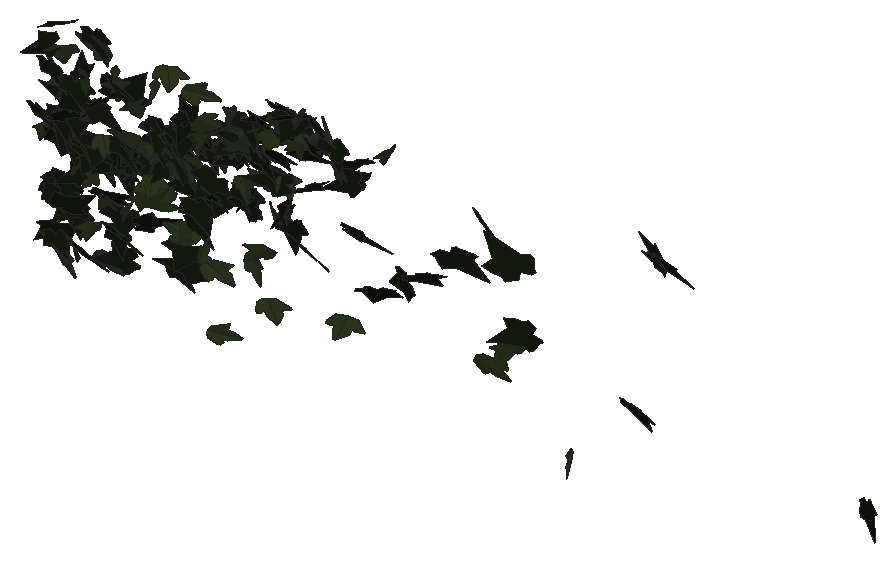
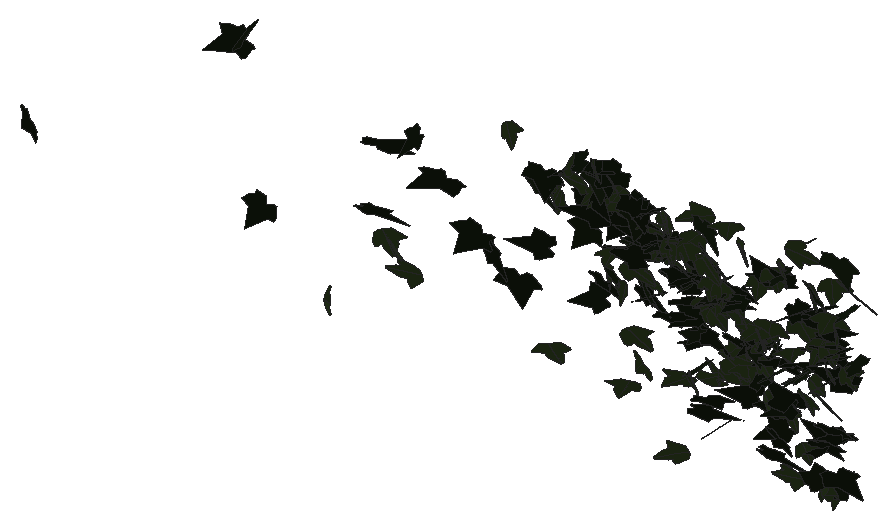
# SketchUp Ruby script. Lengths in millimetres.
U = 1.mm
M = Sketchup.active_model
def pt(a) = Geom::Point3d.new(a.map { |v| v * U })
def face(e, loops, mat)
  f = e.add_face(loops[0].map { |a| pt(a) })
  loops[1..].each { |l| e.add_face(l.map { |a| pt(a) }).erase! }
  f.material = f.back_material = mat if mat
  f
end
# faces: each face lists its corners as indices into pts; further lists are holes
def faces(e, pts, list, mat = nil) = list.each { |f| face(e, (f[0].is_a?(Array) ? f : [f]).map { |l| l.map { |i| pts[i] } }, mat) }
# xy, xz, yz: faces in a plane at the given z, y or x. An outline is a flat list of corners, or four numbers for a rectangle; further outlines are holes
def ring(l) = l.size == 4 ? [[l[0], l[1]], [l[2], l[1]], [l[2], l[3]], [l[0], l[3]]] : l.each_slice(2).to_a
def flat(e, list, mat, &to3) = list.each { |f| face(e, (f[0].is_a?(Array) ? f : [f]).map { |l| ring(l).map { |u, v| to3.(u, v) } }, mat) }
def xy(e, z, list, mat = nil) = flat(e, list, mat) { |x, y| [x, y, z] }
def xz(e, y, list, mat = nil) = flat(e, list, mat) { |x, z| [x, y, z] }
def yz(e, x, list, mat = nil) = flat(e, list, mat) { |y, z| [x, y, z] }
def lines(e, pts, list) = list.each { |a, b| e.add_line(pt(pts[a]), pt(pts[b])) }
# prism: a flat outline (further loops are holes) pulled along v
def prism(e, loops, v, mat = nil)
  f = face(e, loops, mat); d = Geom::Vector3d.new(v.map { |x| x * U })
  f.pushpull(f.normal.samedirection?(d) ? d.length : -d.length)
end
def box(e, o, s, mat = nil) = prism(e, [[o, [o[0] + s[0], o[1], o[2]], [o[0] + s[0], o[1] + s[1], o[2]], [o[0], o[1] + s[1], o[2]]]], [0, 0, s[2]], mat)
def at(x, y, z, deg = 0) = Geom::Transformation.translation(pt([x, y, z])) * Geom::Transformation.rotation(ORIGIN, Z_AXIS, deg.degrees)
def axes(o, x, y, z) = Geom::Transformation.new([*x, 0, *y, 0, *z, 0, *pt(o).to_a, 1])
def part(name) = M.definitions.add(name)
# library, detail: a bought-in or finely detailed component or shape, given as its bounding box
def library(name, o, s) = part(name).tap { |d| box(d.entities, o, s) }
def detail(e, o, s) = box(e.add_group.entities, o, s)
def put(e, d, t, mat = nil) = e.add_instance(d, t).tap { |i| i.material = mat if mat }
def group(e, t, mat = nil) = e.add_group.tap { |g| g.transformation = t; g.material = mat if mat }.entities
root = M.entities
M.materials.add("efeu1").color = [18, 25, 13]
M.materials.add("efeu2").color = [43, 57, 29]
c1 = part("ivyleaf_9")
p = [[39.1,54.8,31.7],[34.5,51.8,30.2],[-5.3,25.2,17.3],[-17.9,28.3,20.9],[-21.6,21.7,17],[-20.2,4.3,5.3],
  [-22.9,-0.3,2.5],[-17.1,-4,-0.6],[-2,-2.1,-1.2],[-0.7,-15.4,-10.1],[16.6,-22.3,-16.7],[21.1,-15.1,-12.5],
  [32.7,-10.7,-11],[46.1,-1.8,-6.6],[30.8,11.2,3.8]]
faces(c1.entities,p,[[0,1,2,3,4,5,6,7,8,9,10,11,12,13,14]],"efeu1")
c2 = part("ivyleaf_10")
p = [[0,12.8,-0.8],[-1.5,51.3,-10.9],[-4.9,51,-11.6],[-13.6,26.5,-7.3],[-13.2,15.9,-4.6],[-21.1,19.3,-7.2],
  [-29.5,16.3,-8.3],[-29.2,8.3,-6.2],[-19.7,-9.8,0.5],[-7.6,-13,4],[1,-12.2,5.8],[-0.4,51.1,-11.1],
  [-1.5,51.1,-10.9],[1,-12.4,5.9],[16.9,-12.4,3.5],[35.1,9.1,-5.1],[35,12.9,-6.1],[20.5,16.4,-4.9],
  [15.8,15,-3.8],[15.3,27.6,-7.1],[12.8,31.3,-7.8]]
faces(c2.entities,p,[[0,1,2,3,4,5,6,7,8,9,10],[11,12,0,13,14,15,16,17,18,19,20]],"efeu2")
put(root,c1,axes([4895,793.5,3135.5],[0.99985,-0.9512,0.16756],[0.29482,-0.10529,-1.0834],[1.81439,0.54128,0.08371]))
put(root,c1,axes([4961.3,784.3,3378.4],[-1.89203,0.5811,-0.0485],[-0.01971,-0.11345,-1.14688],[-1.10962,-0.98882,0.10308]))
put(root,c2,axes([4943.9,791.7,3096.3],[-0.58928,-1.00709,0.34545],[-0.09077,-0.34628,-1.05226],[2.02429,-0.3087,0.05338]))
put(root,c1,axes([4962.2,812,2755.9],[0.28697,0.52098,-0.9616],[-0.43571,-0.93416,-0.54201],[-2.03534,0.27343,-0.01955]))
put(root,c1,axes([4936.5,795.6,3298.9],[0.65973,-1.08228,0.0317],[0.04767,-0.02526,-1.13632],[2.06013,0.34717,0.01614]))
put(root,c1,axes([4984,780.5,3453.5],[0.3733,1.12783,0.06991],[-0.59622,0.12245,-1.09646],[-2.0663,0.16842,0.32901]))
put(root,c1,axes([4958.4,817.5,2889],[-0.64539,-0.93685,-0.37561],[0.2059,0.36022,-0.99614],[1.90991,-0.35541,-0.01953]))
put(root,c1,axes([4941.9,793.4,2697.1],[0.69518,-0.70686,0.73199],[0.65781,-0.6453,-0.79562],[1.82152,0.50281,0.00796]))
put(root,c1,axes([4980.3,824.5,2911.1],[-1.71841,-0.38438,-0.40311],[0.74559,0.10755,-0.98002],[0.75356,-0.98294,0.05041]))
put(root,c2,axes([4982.3,797.2,3233.2],[0.53522,-1.08965,-0.1569],[0.25302,0.19437,-1.11157],[2.07987,0.25676,0.1756]))
put(root,c1,axes([4971.6,788.7,2733.6],[0.1042,-1.05035,-0.32712],[-0.09159,0.32492,-1.05136],[2.09173,0.06655,-0.02974]))
put(root,c1,axes([4941.5,788.9,3060],[0.93088,-0.27009,1.00515],[1.82838,-0.31014,-0.55082],[0.76211,1.07395,0.09372]))
put(root,c1,axes([4973.9,806.5,2878.5],[-0.40069,-1.03674,-0.42166],[0.28163,0.3995,-1.05615],[2.11137,-0.25004,0.06086]))
put(root,c2,axes([5001.1,790.1,3373.3],[-1.33311,-0.90194,-0.06794],[0.08726,0.05042,-1.14198],[1.71922,-0.70194,0.00528]))
put(root,c1,axes([4984.2,793.4,3148],[-0.16469,-1.11858,-0.01331],[-0.00191,0.01343,-1.12192],[2.12903,-0.08651,-0.00204]))
put(root,c2,axes([5007.7,802.8,3161.3],[-0.77688,-1.01331,0.20273],[-0.05131,-0.20746,-1.09122],[1.96609,-0.40581,0.05163]))
put(root,c1,axes([5022.8,818.9,2843],[-1.89321,-0.32974,-0.01532],[0.03036,0.00056,-1.04797],[0.62751,-0.99487,0.00448]))
put(root,c1,axes([4986.9,795,3063.1],[0.94548,-0.73023,-0.66735],[-0.30899,0.67647,-0.86106],[1.85719,0.4843,0.19649]))
put(root,c2,axes([5002.2,797.2,3260.7],[-1.79745,-0.54668,-0.30729],[0.68518,-0.01779,-1.07486],[0.97727,-0.99301,0.18842]))
put(root,c1,axes([5006.1,801.2,3119.2],[-0.90927,-0.95182,0.29186],[-0.12886,-0.29191,-1.06282],[1.89036,-0.47772,0.06794]))
put(root,c1,axes([5026.2,779.8,3169.2],[0.02648,0.89594,-0.78841],[-0.03884,-0.78817,-0.89602],[-2.27102,0.02393,0.00613]))
put(root,c1,axes([5053.2,790.9,3201.9],[-0.25436,0.07532,1.12914],[-1.96334,0.45932,-0.15274],[-0.88544,-1.04012,0.01432]))
put(root,c2,axes([4993.1,793.4,2670.3],[-0.88924,0.53618,-0.86189],[0.95164,-0.70413,-0.7091],[-1.6812,-0.68217,0.05449]))
put(root,c2,axes([5004.3,805.8,3090.8],[1.11525,-0.64936,0.67422],[0.87348,-0.49395,-0.87464],[1.55271,0.74428,0.00776]))
put(root,c2,axes([5003.3,828.6,2686.1],[-0.60815,0.0155,1.03507],[1.43712,-0.73751,0.24415],[1.34769,0.79345,0.20672]))
put(root,c1,axes([5019.3,817.6,2824.3],[-0.42925,-1.06641,-0.15585],[0.10628,0.14745,-1.08973],[2.04839,-0.23112,0.02388]))
put(root,c1,axes([5004.6,781.2,2843.8],[-0.41443,-0.0664,1.09538],[2.07818,0.09809,0.22302],[-0.20797,1.1125,0.04572]))
put(root,c2,axes([5031.2,801.3,3163.3],[-1.16912,-0.93142,-0.56717],[0.59728,0.47243,-1.11575],[1.98767,-0.68981,0.00168]))
put(root,c1,axes([5026.2,812.1,3162.6],[-0.82502,-0.98611,-0.23385],[0.30034,0.18556,-1.07502],[1.90528,-0.45625,0.0682]))
put(root,c1,axes([5023.1,804.4,3069.5],[-0.26273,-1.06103,0.24216],[0.04039,-0.24668,-1.06873],[2.07088,-0.1298,0.05157]))
put(root,c1,axes([5070.2,783.6,2980.5],[-1.66615,0.62673,-0.08734],[0.13592,-0.05029,-1.07666],[-1.19662,-0.87836,-0.00068]))
put(root,c1,axes([5064.8,784.5,3307.3],[0.54372,0.31735,1.06051],[-0.12853,1.09821,-0.31044],[-2.10287,0.01493,0.29318]))
put(root,c1,axes([5047.7,789.7,3274.2],[-0.25318,-1.1131,-0.11797],[0.07277,0.11421,-1.12076],[2.12908,-0.13627,0.02428]))
put(root,c2,axes([5066.7,794.7,3022],[0.05634,-0.93695,0.58434],[0.07367,-0.58331,-0.93726],[2.10027,0.0456,0.0172]))
put(root,c1,axes([5028.4,805,2710.6],[1.3556,-0.62619,0.52452],[0.79045,-0.32162,-0.94796],[1.33866,0.82402,0.0286]))
put(root,c2,axes([5083.4,810.5,2975.3],[1.64045,-0.67832,-0.05307],[-0.08159,0.03133,-1.09684],[1.29236,0.863,-0.00189]))
put(root,c2,axes([5090.5,806.5,2800.7],[-0.74678,-0.94995,0.21409],[0.04261,-0.23956,-1.02191],[1.85279,-0.37737,0.10979]))
put(root,c2,axes([5113.5,796.5,3199.1],[-1.82115,-0.23761,0.53048],[-0.94755,-0.19228,-0.9842],[0.57092,-1.07706,0.05867]))
put(root,c2,axes([5099.6,766.1,3311.6],[0.96397,-0.78962,-0.6812],[-0.38347,0.66893,-0.92521],[1.94735,0.5226,0.15501]))
put(root,c1,axes([5092.1,812.2,3041.7],[-1.05486,-0.86571,0.42191],[-0.01281,-0.4833,-1.00052],[1.83283,-0.50163,0.23583]))
put(root,c1,axes([5080.1,812.5,3050.9],[0.96719,-0.94563,-0.21102],[-0.05406,0.22365,-1.0706],[1.8432,0.50277,0.07933]))
put(root,c1,axes([5108.5,821.3,3081.5],[-1.12385,-0.92501,0.03891],[0.1291,-0.08926,-1.09238],[1.75731,-0.58502,0.10514]))
put(root,c2,axes([5157.6,775.7,3425.3],[-0.14861,0.19579,-1.25186],[-2.04329,0.6559,0.16955],[1.28076,1.06913,0.12524]))
put(root,c1,axes([5139.8,786.8,3247.2],[-0.60774,0.78246,-0.78278],[0.48804,-0.74024,-0.84454],[-2.04913,-0.40837,0.03101]))
put(root,c1,axes([5105.8,825.1,3034.4],[0.46372,-1.06443,-0.00225],[0.00259,0.00262,-1.09196],[2.02583,0.24365,0.00191]))
put(root,c2,axes([5154.9,801.7,2900.8],[-1.54255,0.36473,0.68855],[-1.22178,0.2505,-0.88836],[-0.84045,-1.03357,0.02767]))
put(root,c1,axes([5116.1,786.6,3463.7],[0.23777,-1.14106,-0.07944],[0.03311,0.0818,-1.14758],[2.17666,0.1234,0.02613]))
put(root,c2,axes([5115.1,820.2,2697.9],[-0.83524,0.21107,-0.95915],[1.61639,-0.44597,-0.48674],[-0.93858,-0.95587,0.0153]))
put(root,c2,axes([5139.2,802.4,3106.4],[1.08697,0.9593,-0.02444],[-0.00142,-0.028,-1.11636],[-1.82634,0.57097,-0.01368]))
put(root,c1,axes([5128.1,771.4,3228.5],[0.85114,-0.84391,-0.60624],[0.07189,0.67278,-0.90866],[1.97629,0.33898,0.29415]))
put(root,c1,axes([5137.4,806.3,2918.9],[1.84182,-0.43318,0.00169],[0.08158,0.09165,-1.05544],[0.82038,0.9634,0.10116]))
put(root,c1,axes([5191.7,810.3,3059.6],[-2.03846,-0.19623,0.0523],[-0.10171,0.00146,-1.08884],[0.37289,-1.07234,-0.01106]))
put(root,c1,axes([5138.6,798.7,2921.4],[1.97474,0.33957,-0.26038],[0.47235,0.07878,1.09174],[0.66341,-1.06686,-0.00226]))
put(root,c1,axes([5177.7,821,2808.6],[-1.12659,-0.05492,-0.90653],[1.72743,-0.07337,-0.58823],[-0.06005,-1.08019,0.08604]))
put(root,c1,axes([5235.5,806.3,2736],[-1.83187,0.14666,0.53247],[-0.99706,0.09627,-0.97353],[-0.33278,-1.09577,-0.01426]))
put(root,c2,axes([5200.1,782.1,3358.7],[0.86246,-1.05296,-0.13502],[-0.02913,0.14031,-1.1456],[2.0202,0.45155,0.04112]))
put(root,c1,axes([5175.1,788.6,2830.5],[2.09998,-0.41949,-0.02096],[-0.03264,0.01385,-1.18043],[0.7987,1.10351,0.00685]))
put(root,c1,axes([5191.8,828.6,3016.8],[0.07398,-1.05919,0.23083],[0.11598,-0.22848,-1.05866],[2.0599,0.0509,0.05132]))
put(root,c1,axes([5246,776.7,3092.5],[-0.69455,0.91856,0.47704],[-0.66894,0.36579,-0.97322],[-1.85285,-0.47639,0.17255]))
put(root,c1,axes([5209.2,824.3,3056.2],[-0.91054,-0.97823,-0.09877],[0.09304,0.08604,-1.08894],[1.86893,-0.48088,0.00609]))
put(root,c2,axes([5225.3,786,3331.6],[-1.33233,-0.875,0.19659],[-0.02938,-0.2376,-1.11249],[1.70655,-0.68721,0.13433]))
put(root,c1,axes([5187.9,788.7,3337],[1.14529,-0.96735,-0.0528],[0.16998,0.11728,-1.1309],[1.83594,0.59259,0.13764]))
put(root,c1,axes([5212.8,811.5,3062],[-0.30557,-0.42356,1.01444],[-0.41974,-0.99195,-0.44908],[2.04968,-0.26628,0.05927]))
put(root,c1,axes([5219.8,801.1,2893.8],[-1.49126,-0.6028,-0.38934],[0.56572,0.25205,-0.98845],[1.24307,-0.83786,-0.01723]))
put(root,c2,axes([5229.1,799.6,3157.5],[-2.13061,-0.11384,0.02211],[-0.04337,0.00557,-1.12523],[0.21641,-1.11969,-0.00785]))
put(root,c2,axes([5238.1,819.3,3040],[-0.31358,-1.04964,0.22877],[-0.14572,-0.21938,-1.06171],[2.03937,-0.17707,-0.04069]))
put(root,c2,axes([5232.8,804,2918.1],[0.31779,-1.06075,0.22936],[0.16519,-0.21826,-1.07261],[2.05885,0.18124,0.05066]))
put(root,c1,axes([5216.2,798.1,3125],[0.09227,-1.10628,-0.13717],[0.12569,0.13991,-1.10503],[2.11787,0.0399,0.07156]))
put(root,c1,axes([5227.9,777.2,3296.9],[-1.49566,0.1479,1.03636],[1.94161,-0.18248,0.79964],[0.4469,1.28776,-0.00571]))
put(root,c2,axes([5252.9,816.6,3130.1],[0.7245,-1.03113,0.1237],[0.09716,-0.11301,-1.09912],[1.97414,0.38398,0.0087]))
put(root,c1,axes([5235.6,815.8,3097.3],[0.03295,-0.82058,0.74143],[0.28341,-0.73304,-0.81477],[2.08563,0.11258,0.099]))
put(root,c1,axes([5274.8,824.6,3071.4],[-1.34824,0.4181,-0.72129],[0.76287,-0.65913,-0.77575],[-1.39128,-0.76658,0.27362]))
put(root,c1,axes([5242.8,820.2,2966.5],[-0.11197,-0.52167,0.94009],[0.44356,-0.9253,-0.49888],[1.99754,0.17622,0.16347]))
put(root,c2,axes([5268.7,811.6,3082.4],[-0.03452,0.91133,-0.57721],[-0.45718,-0.5662,-0.88641],[-2.00151,0.11361,0.21242]))
put(root,c2,axes([5279.3,782.9,3286.8],[-1.05418,-0.94917,-0.30611],[0.27077,0.27137,-1.09888],[1.87867,-0.57172,-0.01339]))
put(root,c2,axes([5263.2,816.1,3136.4],[-1.83112,-0.21167,-0.50134],[1.02747,-0.24304,-0.93344],[0.1304,-1.05734,0.31492]))
put(root,c1,axes([5266.3,795.7,3088.1],[0.15876,-0.73778,-0.80673],[0.11525,0.81095,-0.73538],[2.07744,0.01139,0.10245]))
put(root,c2,axes([5297.2,815,2999.3],[1.30859,0.80245,-0.16364],[-0.23494,-0.10968,-1.0565],[-1.54085,0.69822,0.02211]))
put(root,c2,axes([5310.1,786.4,2985.1],[-0.88043,-0.96244,0.09659],[-0.04227,-0.09647,-1.06762],[1.84043,-0.46263,0.02168]))
put(root,c2,axes([5319.4,807.9,3090],[0.62326,-1.02109,-0.106],[0.06065,0.12132,-1.07022],[1.95284,0.32212,0.06707]))
put(root,c1,axes([5338.6,821.1,3083.4],[-1.95326,-0.17049,-0.26648],[0.52006,-0.02192,-1.03838],[0.30337,-1.06011,0.06432]))
put(root,c2,axes([5326.6,796.1,3040.6],[0.95957,0.90977,-0.2903],[-0.34983,-0.22968,-1.03904],[-1.78349,0.53453,0.04762]))
put(root,c1,axes([5297.2,781.8,2889.4],[0.71883,0.2079,1.08516],[1.84758,0.48521,-0.43084],[-1.0042,1.04154,-0.0159]))
put(root,c2,axes([5350.7,822.2,3000],[-1.30393,-0.5885,0.62316],[-0.76408,-0.48451,-0.89896],[1.44127,-0.78929,0.0872]))
put(root,c2,axes([5320.4,808.7,3149.1],[2.03858,-0.30833,0.11835],[0.27071,0.06817,-1.10974],[0.56728,1.07549,0.10428]))
put(root,c2,axes([5337,803.2,3157.6],[1.01887,-0.98347,-0.09124],[-0.10235,0.07461,-1.11967],[1.87698,0.53792,-0.01153]))
put(root,c2,axes([5334,811.8,2949.8],[-1.75351,-0.65919,0.17745],[0.28562,0.0952,1.13284],[-1.26745,0.93344,0.00978]))
put(root,c1,axes([5327,797.2,3216.9],[1.77711,-0.56346,-0.31017],[-0.50477,0.16081,-1.09058],[1.11519,0.97068,0.00063]))
put(root,c2,axes([5353.1,778.9,3372],[0.92115,-1.04479,0.02253],[0.03766,-0.01566,-1.1514],[1.98855,0.48427,0.01137]))
put(root,c2,axes([5363.5,782.9,3175.3],[-1.57263,0.6893,-0.25631],[0.33062,-0.19166,-1.0755],[-1.36001,-0.84365,0.03492]))
put(root,c1,axes([5368.7,794.2,3236.5],[-1.7461,-0.30827,-0.60387],[1.12543,0.13323,-0.96643],[0.63124,-1.09024,0.05265]))
put(root,c1,axes([5368.8,795.9,3224.4],[-1.01141,-0.92833,0.33304],[0.11585,-0.40846,-1.04144],[1.87348,-0.47591,0.24419]))
put(root,c1,axes([5372.4,806.1,3189.7],[-1.3669,-0.77799,-0.32497],[0.52285,0.18766,-1.05642],[1.51709,-0.76565,0.07128]))
put(root,c2,axes([5382.1,781.5,3007.4],[0.19761,-0.51344,0.99573],[-0.33341,0.98025,0.52373],[-2.10594,-0.20337,0.01052]))
put(root,c2,axes([5403.6,807.1,3229.2],[-0.8652,-1.01838,-0.09694],[0.12567,0.07665,-1.11487],[1.94288,-0.45846,0.02894]))
put(root,c2,axes([5389.5,788.6,3434.3],[1.46933,0.84344,-0.02459],[-0.00408,-0.03138,-1.14326],[-1.60591,0.77179,-0.0196]))
put(root,c1,axes([5389.9,817.1,2774.1],[0.73605,-0.94924,-0.42474],[-0.23059,0.40894,-1.02427],[1.96572,0.40341,0.03889]))
put(root,c2,axes([5426.1,809.7,3132.7],[-0.31517,-1.00146,0.40409],[-0.17729,-0.39404,-1.01474],[2.04763,-0.18826,-0.02566]))
put(root,c1,axes([5408.2,817.1,3179.6],[-0.00843,-1.10156,0.03885],[0.00704,-0.03887,-1.10156],[2.09778,-0.0043,0.00385]))
put(root,c2,axes([5430.3,807.2,3235.9],[-1.48822,-0.78736,-0.14111],[0.33168,0.02489,-1.10468],[1.48581,-0.7942,0.10526]))
put(root,c1,axes([5468.1,811.6,3061],[0.0457,-0.02488,-1.08064],[-1.96531,-0.32,-0.01558],[-0.60804,1.03245,-0.03087]))
put(root,c1,axes([5412.9,800.4,3206.2],[1.61601,-0.6193,-0.36403],[-0.42045,0.31119,-1.04469],[1.30095,0.86986,0.11456]))
put(root,c2,axes([5473.9,798.2,3282.3],[-1.24095,0.12835,0.91484],[-1.68063,0.24229,-0.66337],[-0.51639,-1.09698,-0.03948]))
put(root,c2,axes([5463.6,794,2894],[0.86193,0.7039,0.76279],[-1.08702,-0.52589,0.8244],[1.64942,-0.71441,0.1447]))
put(root,c1,axes([5448.2,818.3,2847.5],[-1.51064,-0.77784,0.00642],[-0.01483,-0.00122,-1.11132],[1.48035,-0.79376,-0.00458]))
put(root,c1,axes([5429.8,802.2,3228.1],[-0.37642,-1.00435,0.46953],[0.0362,-0.47994,-1.01862],[2.10974,-0.17096,0.10125]))
put(root,c2,axes([5452.2,783.1,3136.6],[1.76193,-0.49146,-0.36989],[-0.51297,0.27668,-1.04221],[1.05229,0.95777,0.11127]))
put(root,c1,axes([5468.7,785.3,3300.2],[0.0126,0.55795,1.00845],[-0.38389,0.99346,-0.54834],[-2.1596,-0.17334,0.10335]))
put(root,c2,axes([5454.6,801.1,3153.9],[-2.0691,-0.09326,0.04684],[-0.08799,-0.00905,-1.09115],[0.17806,-1.08814,0.00506]))
put(root,c1,axes([5487,812.4,2792.5],[-0.74435,-0.48152,-0.92773],[-1.16664,-0.69666,0.62],[-1.6113,0.72685,-0.02034]))
put(root,c1,axes([5449.2,802.5,3159.2],[-0.87527,-1.03339,-0.02298],[-0.00379,0.02603,-1.13103],[1.96722,-0.45973,-0.0124]))
put(root,c2,axes([5461,778.8,2932.6],[1.50211,-0.81529,-0.0645],[-0.04077,0.069,-1.13427],[1.55597,0.78887,0.03255]))
put(root,c1,axes([5461.8,787,3295.8],[-1.65366,0.24812,-0.71186],[1.32202,-0.15856,-0.90312],[-0.55748,-1.11201,-0.03006]))
put(root,c1,axes([5493.5,779.1,3400.9],[-0.53039,1.11691,0.13877],[-0.00223,0.14267,-1.15067],[-2.14204,-0.27671,-0.03316]))
put(root,c1,axes([5463.9,820.2,2946.5],[0.72763,-0.99158,-0.21043],[-0.08668,0.20787,-1.06226],[1.92725,0.38371,0.03167]))
put(root,c1,axes([5470.6,826.3,3058.9],[0.87932,-0.94385,0.29757],[0.2337,-0.27119,-1.05083],[1.86894,0.47798,-0.0086]))
put(root,c1,axes([5492.4,800.6,3016.8],[-0.48129,-0.98758,-0.43939],[0.41216,0.39581,-1.01428],[2.01549,-0.31677,0.10249]))
put(root,c2,axes([5515,793.8,2847.2],[1.45026,-0.89613,0.14041],[-0.17351,0.10679,1.17631],[-1.71758,-0.76745,-0.00027]))
put(root,c1,axes([5502.1,821,3213.3],[0.43088,-1.07078,0.10416],[0.04274,-0.10172,-1.09445],[2.04708,0.22751,0.00093]))
put(root,c1,axes([5560.1,791.1,3209.4],[-0.25716,0.56337,0.94543],[-1.18614,0.74591,-0.53355],[-1.72637,-0.59641,0.22576]))
put(root,c2,axes([5533.3,787.5,3265.2],[-0.12446,-1.01073,0.46922],[0.10348,-0.47236,-1.00992],[2.11827,-0.03631,0.07691]))
put(root,c2,axes([5502.5,758.4,3416.9],[0.54575,0.23435,1.15344],[1.06827,1.01626,-0.34602],[-1.96894,0.61634,0.13197]))
put(root,c1,axes([5520.4,821.4,3222.9],[-0.31824,-1.05797,-0.24772],[-0.00383,0.25094,-1.07035],[2.06798,-0.16235,-0.04011]))
put(root,c2,axes([5543.1,800.8,3305.4],[-0.73289,-1.04047,0.20579],[0.01205,-0.22118,-1.10646],[2.01854,-0.37645,0.08132]))
put(root,c1,axes([5494,811.2,3207.5],[1.19683,-0.44126,0.80937],[1.23975,-0.48056,-0.76811],[1.24142,0.90532,-0.01323]))
put(root,c1,axes([5516.5,777.1,3087.9],[2.04751,-0.17845,-0.0565],[-0.10494,0.01285,-1.09052],[0.34043,1.07723,0.00365]))
put(root,c1,axes([5559.2,797.1,3128.8],[-1.3612,-0.82021,0.27547],[-0.35303,-0.20373,-1.08823],[1.60842,-0.73886,-0.00573]))
put(root,c2,axes([5538,763.5,3331.1],[-0.88553,-0.6187,-0.89971],[1.10933,0.68625,-0.77334],[1.75725,-0.745,0.03482]))
put(root,c1,axes([5540.2,818.5,3234.2],[-1.08082,-0.59905,-0.72963],[0.90292,0.55505,-0.82497],[1.55335,-0.73945,-0.02815]))
put(root,c2,axes([5575.2,790.6,3220.5],[-1.26478,0.88841,0.028],[-0.02496,0.02515,-1.10945],[-1.69147,-0.66467,-0.00456]))
put(root,c1,axes([5607.3,784.7,3316.3],[-0.19577,1.06931,-0.33204],[-0.51105,-0.34727,-1.03516],[-2.06879,-0.0154,0.28714]))
put(root,c1,axes([5587.7,819,3079.8],[-1.48093,-0.76443,-0.08932],[0.08823,0.08024,-1.09051],[1.46209,-0.77911,-0.02467]))
put(root,c2,axes([5563.9,794.6,2612.4],[0.47426,0.22073,1.11663],[0.83119,1.03704,-0.30246],[-2.00048,0.48322,0.13905]))
put(root,c2,axes([5600.2,804.8,3305.6],[-0.66777,-1.06359,-0.0843],[0.02264,0.08483,-1.11987],[2.03045,-0.35074,-0.01523]))
put(root,c2,axes([5605.4,811.7,3300.1],[-2.05886,0.25748,0.11079],[-0.28961,-0.16852,-1.09421],[-0.44803,-1.07431,0.1982]))
put(root,c2,axes([5574.8,766,2847.5],[1.12174,0.63968,0.77751],[1.06628,0.54019,-0.86914],[-1.59213,0.81247,-0.03428]))
put(root,c2,axes([5633.5,783.3,3368.3],[-1.54001,0.71764,0.32519],[-0.77233,0.01994,-1.05377],[-1.2853,-0.87184,0.24357]))
put(root,c1,axes([5596.8,796,3284.3],[1.27017,-0.89287,0.00332],[0.00384,-0.00264,-1.11473],[1.69933,0.66739,0.00004]))
put(root,c2,axes([5630.4,793.7,3374.9],[0.62446,-1.08627,-0.10958],[0.0186,0.11734,-1.13392],[2.0778,0.32542,0.04309]))
put(root,c1,axes([5652.3,797.8,3290.4],[-1.77035,-0.55,0.25967],[-0.20316,-0.3195,-1.05911],[1.13959,-0.91138,0.21459]))
put(root,c1,axes([5629.8,807.9,3306.4],[-0.51063,-1.0801,-0.10082],[0.05823,0.09628,-1.11291],[2.06376,-0.26996,0.00646]))
put(root,c1,axes([5669.2,779.4,3254.4],[-1.85926,0.52652,-0.06574],[0.1086,-0.03268,-1.10976],[-1.004,-0.97857,0.00169]))
put(root,c2,axes([5648.1,773.9,3278.5],[-2.06053,-0.24176,-0.06386],[0.12207,0.00577,-1.1093],[0.45998,-1.08453,0.00833]))
put(root,c2,axes([5666.7,783.3,3278.5],[-0.61024,-1.03118,0.231],[-0.20239,-0.20869,-1.07918],[2.00097,-0.33559,-0.0387]))
put(root,c1,axes([5687.5,811.2,3129.3],[-1.33889,0.54739,-0.66374],[1.03921,-0.37849,-0.89089],[-1.26535,-0.89005,-0.02936]))
put(root,c1,axes([5663.9,818,3112.8],[-0.18849,-1.09832,-0.04645],[0.17375,0.03826,-1.0993],[2.08496,-0.10248,0.08741]))
put(root,c2,axes([5672.6,807.7,3328.2],[2.10155,0.10414,0.03894],[0.07272,0.0096,-1.1091],[-0.19871,1.10486,0.00596]))
put(root,c1,axes([5720.9,778.9,3100.1],[-0.3131,0.03207,-1.14396],[-2.17722,-0.03628,0.1635],[-0.05968,1.15516,0.03689]))
put(root,c2,axes([5679.2,799.7,3282.1],[1.9815,-0.37727,-0.00631],[0.11882,0.19051,-1.08911],[0.70823,1.02358,0.20038]))
put(root,c2,axes([5662.4,797.9,3155.4],[1.45914,-0.48593,0.67987],[1.13488,-0.32829,-0.90708],[1.11426,0.97069,0.03357]))
put(root,c1,axes([5641.6,812.1,3302.7],[1.01026,-0.13605,0.96901],[1.78161,-0.25041,-0.54796],[0.5423,1.07613,-0.005]))
put(root,c1,axes([5649.8,811.5,3300.2],[1.47001,-0.70065,0.39286],[0.63928,-0.21336,-1.0409],[1.38871,0.83988,0.06331]))
put(root,c2,axes([5691.7,806.6,3327.9],[-0.79352,-0.94867,0.42173],[0.2065,-0.49179,-0.99901],[1.96505,-0.33141,0.27528]))
put(root,c2,axes([5694.5,785.4,3316.5],[-0.71043,-1.03666,-0.34856],[0.25391,0.32239,-1.10171],[2.06596,-0.3961,0.01554]))
put(root,c1,axes([5691.1,792.2,3373.1],[-0.22055,-1.13441,-0.04033],[-0.02258,0.04175,-1.1402],[2.16025,-0.11538,-0.01603]))
put(root,c2,axes([5743.7,810.5,3178.5],[-1.05376,-0.26675,0.92514],[-1.59233,-0.39484,-0.61457],[0.90685,-1.00327,-0.00411]))
put(root,c2,axes([5683,824.5,2877.7],[1.4211,-0.57144,0.76372],[1.30712,-0.35094,-0.93407],[1.25972,1.00879,0.10766]))
put(root,c2,axes([5704.3,796.5,3348.9],[-0.54825,0.89779,-0.59532],[0.36437,-0.56376,-0.94283],[-2.01755,-0.34578,-0.0085]))
put(root,c1,axes([5722.7,795.3,3353.7],[0.6025,1.03061,0.29479],[0.1245,0.28823,-1.07792],[-2.03631,0.32256,0.02132]))
put(root,c1,axes([5730.6,795.7,3396.5],[0.56255,1.03464,-0.3641],[-0.21994,-0.34561,-1.07593],[-2.07588,0.317,0.01533]))
put(root,c2,axes([5746.3,797,2951],[-1.05201,-0.71768,0.69491],[-0.84307,-0.53575,-0.90567],[1.70412,-0.7081,-0.01907]))
put(root,c1,axes([5698.1,812.1,3223.6],[1.29731,-0.32808,0.8159],[1.42904,-0.32021,-0.75607],[0.8712,1.0138,0.02523]))
put(root,c1,axes([5727.8,788.1,3274.8],[0.75927,-1.03519,0.054],[0.05761,-0.0462,-1.10934],[1.97201,0.39992,0.01162]))
put(root,c1,axes([5723.2,797.3,3377.8],[1.14985,-0.62119,0.73345],[0.97432,-0.52523,-0.86654],[1.54821,0.7919,0.0006]))
put(root,c2,axes([5778,798.4,3097.6],[-1.25321,0.85347,0.28196],[-0.43566,0.17878,-1.0757],[-1.65426,-0.69364,0.06969]))
put(root,c2,axes([5763,798.7,2775.8],[1.49797,0.74633,0.28902],[0.35598,0.2226,-1.0842],[-1.48102,0.80838,0.03172]))
put(root,c1,axes([5821.1,795.5,3201.4],[-1.43646,0.11676,0.82524],[-1.58621,-0.1122,-0.74639],[0.00921,-1.1127,0.16185]))
put(root,c2,axes([5794,786.7,3361.1],[1.39362,0.74241,-0.40554],[-0.81359,-0.1381,-1.0247],[-1.38932,0.82558,0.19327]))
put(root,c1,axes([5787.7,773.6,3309.4],[2.02812,0.19764,-0.26871],[-0.51921,-0.00121,-1.08278],[-0.36531,1.09899,0.04713]))
put(root,c2,axes([5796.9,790.4,3411.7],[-1.80802,0.48872,-0.35756],[0.45703,-0.30662,-1.05711],[-1.05799,-0.96763,0.15438]))
put(root,c2,axes([5814,805.3,3206],[0.68155,1.03504,0.25044],[-0.00211,0.26458,-1.09191],[-2.02673,0.34779,0.08535]))
put(root,c1,axes([5807.8,782.6,3465.3],[2.15572,-0.04449,-0.16027],[-0.30007,0.06435,-1.13209],[0.10088,1.14215,0.05754]))
put(root,c1,axes([5839.6,795,3134.4],[-1.43933,0.41017,-0.71675],[1.04111,-0.47925,-0.85146],[-1.1774,-0.92519,0.1233]))
put(root,c2,axes([5835.9,799.7,3127.1],[0.59561,-1.05852,0.16082],[0.41117,-0.10167,-1.08962],[1.99579,0.33684,0.17649]))
put(root,c2,axes([5819.8,798.7,3417.4],[0.89961,-0.57451,-0.85162],[1.04379,-0.65154,0.74395],[-1.65319,-0.724,0.00629]))
put(root,c1,axes([5862.1,771.1,3454.7],[0.75963,1.04476,-0.16517],[-0.19021,-0.13849,-1.11756],[-2.00408,0.40916,0.04347]))
put(root,c1,axes([5871,791.3,3439.1],[-1.57974,-0.77358,0.01734],[-0.02828,-0.00949,-1.13463],[1.47237,-0.83017,-0.00319]))
put(root,c1,axes([5856.2,790.7,3085.1],[-1.37123,-0.06467,-0.89539],[1.70586,0.01255,-0.72213],[0.09579,-1.1492,0.0425]))
put(root,c1,axes([5889.4,790.2,3413.8],[0.13565,0.98424,0.54845],[-0.26414,0.55303,-0.97442],[-2.12806,-0.00591,0.15591]))
put(root,c1,axes([5909.7,797.7,3370.1],[0.54292,0.44154,-0.99676],[-1.91313,-0.29223,-0.41714],[-0.80303,0.99474,0.31989]))
put(root,c2,axes([5885.5,795.7,3456.7],[0.62442,-1.0767,0.15848],[0.06535,-0.1552,-1.12551],[2.07022,0.32965,-0.01227]))
put(root,c2,axes([5887.5,779.7,3359],[0.43403,-0.42079,-1.03271],[0.43959,1.04905,-0.37645],[2.07633,-0.13414,0.29557]))
put(root,c2,axes([5882.2,782,3373.1],[-0.75755,-0.6389,-0.85217],[0.98588,0.67876,-0.75085],[1.77115,-0.65109,0.05346]))
put(root,c1,axes([5851.8,807.3,3311.2],[1.46457,-0.17255,0.79377],[1.54397,0.10734,-0.76314],[0.07905,1.10033,0.19893]))
put(root,c1,axes([5856.7,795.6,3027.4],[1.85836,-0.7129,0.23758],[0.37222,-0.13503,-1.20898],[1.38086,0.99582,0.00615]))
put(root,c1,axes([5918.3,776.7,3232.9],[1.04379,0.8665,0.47006],[0.47611,0.39797,-1.02548],[-1.81474,0.6028,0.00133]))
put(root,c1,axes([5943.1,780.9,3455.7],[1.58469,-0.70813,-0.30782],[-0.38843,0.23475,-1.09212],[1.41727,0.85612,0.04486]))
put(root,c2,axes([5939.5,799.1,3388],[-0.52704,0.10001,-1.09155],[1.58585,-0.71226,-0.27665],[-1.35537,-0.87227,0.10075]))
put(root,c2,axes([5991.7,793.3,3420.9],[-0.8589,1.01792,-0.24488],[-0.15568,0.23156,1.11332],[1.98649,0.45826,-0.01863]))
put(root,c2,axes([6020.1,797,3319.5],[-1.49518,0.81372,0.11055],[-0.37392,-0.0377,-1.11872],[-1.51751,-0.79246,0.16674]))
put(root,c1,axes([6005,792,3407.6],[-0.07564,-1.14103,-0.01509],[0.00126,0.01508,-1.14172],[2.1718,-0.03975,0.00014]))
put(root,c2,axes([6025.7,791.4,3338.5],[-0.39236,1.11368,-0.15147],[0.03254,-0.15088,-1.13255],[-2.13882,-0.2066,0.01055]))
put(root,c2,axes([6037,812.6,2808.8],[1.66901,0.72816,-0.40792],[-0.62893,-0.24042,-1.13959],[-1.45867,0.93682,0.02461]))
put(root,c1,axes([6081.3,788.4,3371.2],[0.81822,1.05413,-0.14889],[-0.12831,-0.1333,-1.13837],[-2.02207,0.43501,0.01198]))
put(root,c1,axes([6108.9,774.1,3317.5],[-1.8719,0.57281,0.12129],[-0.19934,0.06117,-1.1382],[-1.09637,-0.98912,-0.00015]))
put(root,c1,axes([6128.9,781.1,3319.6],[-1.25979,0.92991,-0.07281],[0.07559,-0.0611,-1.14144],[-1.77362,-0.66312,0.00307]))
put(root,c1,axes([6066.6,799.3,3129.4],[1.61306,-0.44388,0.65956],[1.17783,-0.23681,-0.95463],[0.94979,1.04751,0.06367]))
put(root,c1,axes([6183,779.2,2979.8],[1.16125,0.8973,-0.42177],[-0.54199,-0.31576,-1.08376],[-1.80748,0.67117,0.054]))
put(root,c2,axes([6227.7,777.3,3464.4],[-0.32893,-1.14447,-0.10702],[0.00828,0.10757,-1.15738],[2.18764,-0.17249,-0.01171]))
put(root,c1,axes([6289.2,785.4,3040.6],[0.28277,0.01202,-1.22368],[-2.30246,0.18708,-0.14505],[0.35075,1.21839,0.03434]))
put(root,c1,axes([6330.1,781.8,3076.1],[1.70091,0.78416,0.33838],[0.43792,0.25059,-1.18844],[-1.56533,0.92218,0.03521]))
put(root,c1,axes([6472.5,769.2,3205.8],[-0.28966,-0.23715,-1.21814],[1.26109,1.02216,-0.28179],[1.99704,-0.67987,0.00126]))
put(root,c1,axes([6546.7,804.8,3340.3],[1.69258,-0.54395,-0.59762],[-0.98212,0.30161,-1.04245],[1.18359,1.02815,-0.01037]))
put(root,c2,axes([6567.8,798.2,2865.3],[-0.80578,0.21866,-1.1022],[1.93053,-0.43238,-0.47542],[-0.9201,-1.0987,-0.03227]))
put(root,c2,axes([6630.7,794.5,2904.8],[1.04272,-0.86317,-0.64065],[0.87351,-0.46238,1.01549],[-1.84997,-0.70485,0.11839]))
put(root,c2,axes([6677.5,793.9,2954.1],[-1.15237,-1.0178,0.25521],[-0.24418,-0.22062,-1.18428],[1.98206,-0.61893,0.00248]))
put(root,c1,axes([6713,777.7,3233.8],[-2.48832,-0.60904,-0.07192],[-0.12153,-0.03323,1.44233],[-1.16083,1.30899,0.00315]))
put(root,c1,axes([6745.7,793,3020.9],[-2.12533,-0.15173,0.4622],[-0.86011,-0.10474,-1.12627],[0.34265,-1.20404,0.03972]))
put(root,c2,axes([6891.7,798.9,2658.6],[0.47707,-0.66036,1.01602],[1.02264,-0.86938,-0.69762],[2.06711,0.58251,0.11063]))
put(root,c1,axes([7119.8,803.6,2905.8],[2.21204,-0.16369,-0.46715],[-0.88355,0.0532,-1.17369],[0.32687,1.25151,-0.01121]))
put(root,c1,axes([7217.4,818.6,3419.5],[0.16879,-1.24031,0.50443],[0.15694,0.50964,1.23862],[-2.54349,-0.05086,0.1099]))
put(root,c1,axes([7198.6,810.3,3432.7],[2.43481,-0.37984,0.13419],[0.23735,-0.05139,-1.33445],[0.72902,1.28531,-0.0137]))
put(root,c1,axes([8002.3,807.2,2880.3],[-0.80287,0.13257,-1.2627],[2.31621,-0.3369,-0.44196],[-0.68849,-1.28797,-0.01436]))
